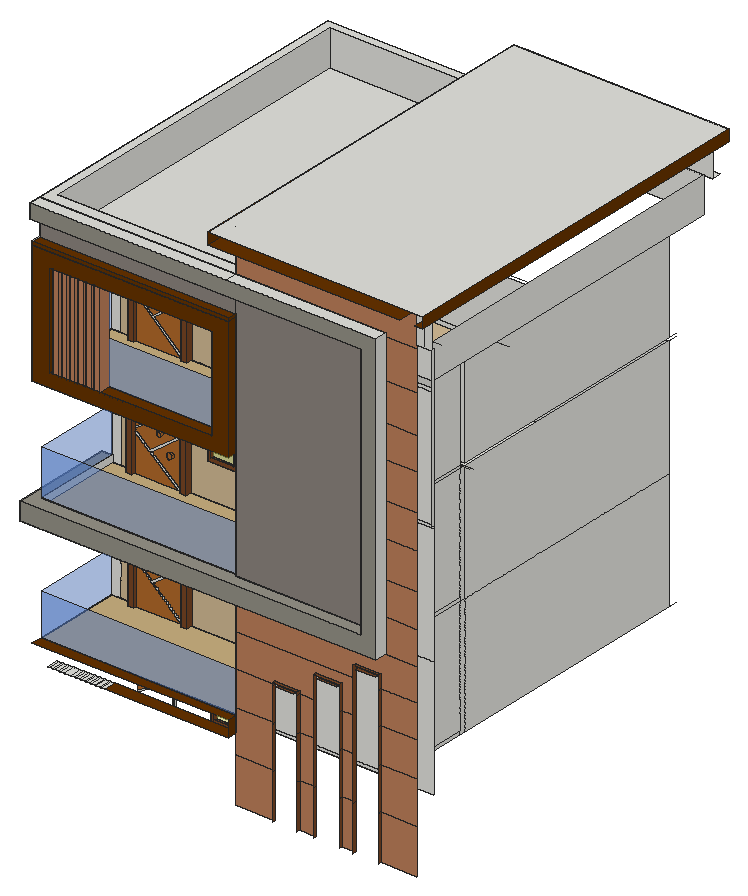
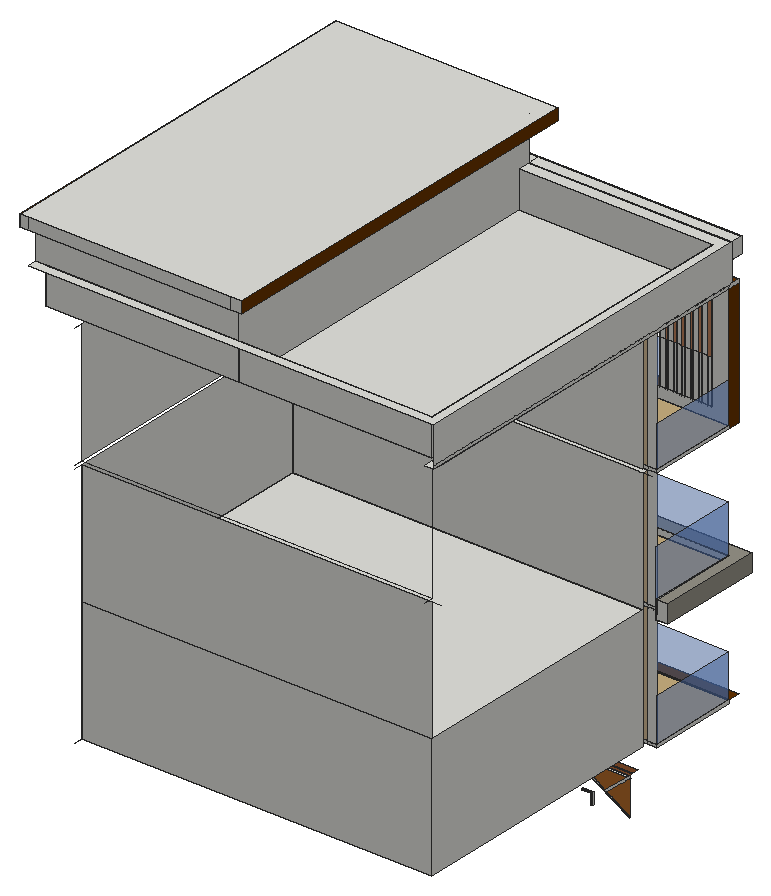
# SketchUp Ruby script. Lengths in inches.
U = 1.inch
M = Sketchup.active_model
def pt(a) = Geom::Point3d.new(a.map { |v| v * U })
def face(e, loops, mat)
  f = e.add_face(loops[0].map { |a| pt(a) })
  loops[1..].each { |l| e.add_face(l.map { |a| pt(a) }).erase! }
  f.material = f.back_material = mat if mat
  f
end
# faces: each face lists its corners as indices into pts; further lists are holes
def faces(e, pts, list, mat = nil) = list.each { |f| face(e, (f[0].is_a?(Array) ? f : [f]).map { |l| l.map { |i| pts[i] } }, mat) }
# xy, xz, yz: faces in a plane at the given z, y or x. An outline is a flat list of corners, or four numbers for a rectangle; further outlines are holes
def ring(l) = l.size == 4 ? [[l[0], l[1]], [l[2], l[1]], [l[2], l[3]], [l[0], l[3]]] : l.each_slice(2).to_a
def flat(e, list, mat, &to3) = list.each { |f| face(e, (f[0].is_a?(Array) ? f : [f]).map { |l| ring(l).map { |u, v| to3.(u, v) } }, mat) }
def xy(e, z, list, mat = nil) = flat(e, list, mat) { |x, y| [x, y, z] }
def xz(e, y, list, mat = nil) = flat(e, list, mat) { |x, z| [x, y, z] }
def yz(e, x, list, mat = nil) = flat(e, list, mat) { |y, z| [x, y, z] }
def lines(e, pts, list) = list.each { |a, b| e.add_line(pt(pts[a]), pt(pts[b])) }
# prism: a flat outline (further loops are holes) pulled along v
def prism(e, loops, v, mat = nil)
  f = face(e, loops, mat); d = Geom::Vector3d.new(v.map { |x| x * U })
  f.pushpull(f.normal.samedirection?(d) ? d.length : -d.length)
end
def box(e, o, s, mat = nil) = prism(e, [[o, [o[0] + s[0], o[1], o[2]], [o[0] + s[0], o[1] + s[1], o[2]], [o[0], o[1] + s[1], o[2]]]], [0, 0, s[2]], mat)
def at(x, y, z, deg = 0) = Geom::Transformation.translation(pt([x, y, z])) * Geom::Transformation.rotation(ORIGIN, Z_AXIS, deg.degrees)
def axes(o, x, y, z) = Geom::Transformation.new([*x, 0, *y, 0, *z, 0, *pt(o).to_a, 1])
def part(name) = M.definitions.add(name)
# library, detail: a bought-in or finely detailed component or shape, given as its bounding box
def library(name, o, s) = part(name).tap { |d| box(d.entities, o, s) }
def detail(e, o, s) = box(e.add_group.entities, o, s)
def put(e, d, t, mat = nil) = e.add_instance(d, t).tap { |i| i.material = mat if mat }
def group(e, t, mat = nil) = e.add_group.tap { |g| g.transformation = t; g.material = mat if mat }.entities
root = M.entities
M.materials.add("[Color C08]").color = [102, 51, 0]
M.materials.add("[Concrete Scored Jointless]").color = [140, 133, 127]
M.materials.add("[Formica Beige]").color = [211, 187, 149]
M.materials.add("[Formica Graystone]").color = [149, 146, 135]
M.materials.add("[Roofing Slate Tan]").color = [200, 175, 128]
M.materials.add("[Translucent Glass Blue]").color = [100, 149, 237]
M.materials["[Translucent Glass Blue]"].alpha = 0.5
M.materials.add("[Translucent Glass Gray]").color = [208, 209, 80]
M.materials["[Translucent Glass Gray]"].alpha = 0.5
M.materials.add("[Wood Bamboo]").color = [177, 105, 43]
M.materials.add("[Wood Veneer 01]").color = [120, 70, 37]
M.materials.add("[Wood Veneer 02]").color = [190, 128, 91]
prism(root,[[[75.279,109.4375,168.805],[75.279,109.4375,179.68],[85.654,109.4375,179.68],[85.654,109.4375,178.68],[76.654,109.4375,178.68],[76.654,109.4375,168.805]]],[0,-1,0])
xy(root,168.023,[[112.818,109.4375,168.881,112.4375]],"[Wood Veneer 01]")
xy(root,171.023,[[115.818,109.4375,135.318,112.4375],[138.318,109.4375,165.881,112.4375]],"[Wood Veneer 01]")
xy(root,207,[[39.278,109.4375,87.278,112.4375]])
xy(root,207,[[39.278,106.4375,87.278,109.4375]],"[Wood Veneer 01]")
xy(root,213,[[33.278,106.4375,93.278,112.4375]],"[Wood Veneer 01]")
xy(root,215.398,[[115.818,109.4375,135.318,112.4375],[138.318,109.4375,165.881,112.4375]],"[Wood Veneer 01]")
xy(root,218.398,[[112.818,109.4375,168.881,112.4375]],"[Wood Veneer 01]")
xy(root,230.125,[[43.358,12.4375,47.175,24.4375]])
xy(root,230.447,[[25.478,12.4375,27.42,24.4375],[27.42,12.4375,31.237,24.4375],[31.237,12.4375,32.733,24.4375],[32.733,12.4375,36.55,24.4375],[36.55,12.4375,38.045,24.4375],
  [38.045,12.4375,41.862,24.4375],[41.862,12.4375,48.67,24.4375],[48.67,12.4375,52.487,24.4375],[52.487,12.4375,53.983,24.4375],[53.983,12.4375,57.8,24.4375],
  [57.8,12.4375,59.295,24.4375],[59.295,12.4375,63.112,24.4375],[63.112,12.4375,64.358,24.4375],[64.358,12.4375,68.175,24.4375],[68.175,12.4375,69.42,24.4375],
  [69.42,12.4375,73.237,24.4375],[73.237,12.4375,74.483,24.4375],[74.483,12.4375,78.3,24.4375],[78.3,12.4375,79.545,24.4375],[79.545,12.4375,83.362,24.4375]])
xy(root,230.447,[[83.362,12.4375,207.712,24.4375]],"[Color C08]")
xy(root,243,[[19.125,118.4375,361.125,375.4375]])
xy(root,243,[[19.125,24.4375,361.125,112.4375]],"[Formica Beige]")
xy(root,246,[[207.712,21.4375,207.712,24.4375,10.125,24.4375],[30.863,106.4375,36.863,112.4375],[84.863,106.4375,90.863,112.4375],[36.863,109.4375,84.863,112.4375]])
xy(root,246,[[10.125,12.4375,207.712,12.4375,207.712,21.4375,10.125,24.4375]],"[Color C08]")
xy(root,246,[[10.125,24.4375,361.125,24.4375,361.125,112.4375,90.863,112.4375,90.863,106.4375,84.863,106.4375,84.863,109.4375,36.863,109.4375,36.863,106.4375,30.863,106.4375,30.863,112.4375,10.125,112.4375]],"[Roofing Slate Tan]")
xy(root,287.148,[[110.131,109.4375,166.193,112.4375]],"[Wood Veneer 01]")
xy(root,288.381,[[250.532,18.4375,269.237,21.4375]],"[Wood Veneer 01]")
xy(root,290.148,[[113.131,109.4375,135.318,112.4375],[138.318,109.4375,163.193,112.4375]],"[Wood Veneer 01]")
xy(root,291.381,[[247.532,18.4375,272.237,21.4375]],"[Wood Veneer 01]")
xy(root,309.988,[[291.733,18.4375,311.736,21.4375]],"[Wood Veneer 01]")
xy(root,312.988,[[288.733,18.4375,314.736,21.4375]],"[Wood Veneer 01]")
xy(root,330,[[36.863,106.4375,84.863,109.4375]])
xy(root,332.471,[[331.649,18.4375,351.153,21.4375]],"[Wood Veneer 01]")
xy(root,334.523,[[113.131,109.4375,135.318,112.4375],[138.318,109.4375,163.193,112.4375]],"[Wood Veneer 01]")
xy(root,335.471,[[328.649,18.4375,354.153,21.4375]],"[Wood Veneer 01]")
xy(root,336,[[30.863,106.4375,90.863,112.4375]],"[Wood Veneer 01]")
xy(root,337.523,[[110.131,109.4375,166.193,112.4375]],"[Wood Veneer 01]")
xy(root,354.75,[[0,9.4375,0,112.4375,10.785,112.4375,10.785,23.9375,207.712,23.9375,207.712,21.4375,343.389,21.4375,343.389,9.4375],[343.389,9.4375,358.6875,21.4375]],"[Formica Graystone]")
xy(root,363,[[19.125,118.4375,361.125,375.4375]])
xy(root,363,[[10.125,24.4375,361.125,112.4375]],"[Formica Beige]")
xy(root,366,[[29.633,106.4375,35.633,112.4375],[83.633,106.4375,89.633,112.4375],[35.633,109.4375,83.633,112.4375]])
xy(root,366,[[10.125,24.4375,361.125,24.4375,361.125,112.4375,89.633,112.4375,89.633,106.4375,83.633,106.4375,83.633,109.4375,35.633,109.4375,35.633,106.4375,29.633,106.4375,29.633,112.4375,10.125,112.4375]],"[Roofing Slate Tan]")
xy(root,372.201,[[0,9.4375,343.389,9.4375,343.389,21.4375,207.712,21.4375,207.712,23.9375,10.785,23.9375,10.785,112.4375,0,112.4375]],"[Formica Graystone]")
xy(root,403.273,[[109.068,109.4375,171.131,112.4375]])
xy(root,406.273,[[112.068,109.4375,135.318,112.4375],[138.318,109.4375,168.131,112.4375]],"[Wood Veneer 01]")
xy(root,450,[[35.633,106.4375,83.633,109.4375]])
xy(root,456,[[29.633,106.4375,89.633,112.4375]],"[Wood Veneer 01]")
xy(root,456.648,[[112.068,109.4375,135.318,112.4375],[138.318,109.4375,168.131,112.4375]],"[Wood Veneer 01]")
xy(root,459.648,[[109.068,109.4375,171.131,112.4375]],"[Wood Veneer 01]")
xy(root,483,[[19.125,112.4375,361.125,118.4375]])
xy(root,483,[[10.125,12.4375,207.712,24.4375]],"[Color C08]")
xy(root,483,[[10.125,24.4375,361.125,112.4375]],"[Formica Beige]")
xy(root,486,[[30.871,106.4375,36.871,112.4375],[84.871,106.4375,90.871,112.4375],[36.871,109.4375,84.871,112.4375]])
xy(root,486,[[10.125,24.4375,361.125,24.4375,361.125,112.4375,90.871,112.4375,90.871,106.4375,84.871,106.4375,84.871,109.4375,36.871,109.4375,36.871,106.4375,30.871,106.4375,30.871,112.4375,10.125,112.4375]],"[Roofing Slate Tan]")
xy(root,496.354,[[31.283,12.4375,37.045,24.4375],[37.045,12.4375,39.47,24.4375],[39.47,12.4375,45.233,24.4375],[45.233,12.4375,47.658,24.4375],[47.658,12.4375,53.42,24.4375],
  [53.42,12.4375,55.845,24.4375],[55.845,12.4375,61.608,24.4375],[61.608,12.4375,64.033,24.4375],[64.033,12.4375,69.795,24.4375],[69.795,12.4375,72.22,24.4375],
  [72.22,12.4375,77.983,24.4375]])
xy(root,496.354,[[27.41,12.4375,31.283,24.4375],[77.983,12.4375,190.722,24.4375]],"[Color C08]")
xy(root,525.398,[[110.131,109.4375,166.193,112.4375]],"[Wood Veneer 01]")
xy(root,528.398,[[113.131,109.4375,135.318,112.4375],[138.318,109.4375,163.193,112.4375]],"[Wood Veneer 01]")
xy(root,536.456,[[60.026,108.4375,74.714,109.4375]],"[Wood Bamboo]")
xy(root,540.894,[[60.026,108.4375,74.714,109.4375]],"[Wood Bamboo]")
xy(root,570,[[36.871,106.4375,84.871,109.4375]])
xy(root,572.773,[[113.131,109.4375,135.318,112.4375],[138.318,109.4375,163.193,112.4375]])
xy(root,575.773,[[110.131,109.4375,166.193,112.4375]])
xy(root,576,[[30.871,106.4375,90.871,112.4375]],"[Wood Veneer 01]")
xy(root,591.0625,[[27.41,12.4375,31.283,24.4375],[31.283,12.4375,37.045,24.4375],[37.045,12.4375,39.47,24.4375],[39.47,12.4375,45.233,24.4375],[45.233,12.4375,47.658,24.4375],
  [47.658,12.4375,53.42,24.4375],[53.42,12.4375,55.845,24.4375],[55.845,12.4375,61.608,24.4375],[61.608,12.4375,64.033,24.4375],[64.033,12.4375,69.795,24.4375],
  [69.795,12.4375,72.22,24.4375],[72.22,12.4375,77.983,24.4375]])
xy(root,591.0625,[[77.983,12.4375,190.722,24.4375]],"[Color C08]")
xy(root,606,[[10.125,12.4375,207.712,24.4375],[10.125,118.4375,19.125,375.4375],[10.125,375.4375,19.125,384.4375]])
xy(root,606,[[10.125,24.4375,361.125,112.4375]],"[Formica Beige]")
xy(root,609,[[10.125,21.4375,207.712,24.4375],[19.125,33.4375,207.712,375.4375]])
xy(root,609,[[10.125,12.4375,207.712,21.4375]],"[Color C08]")
xy(root,630.0625,[[10.125,9.4375,207.712,21.4375],[207.712,9.4375,343.389,21.4375]])
xy(root,645,[[10.125,9.4375,207.712,21.4375],[207.712,9.4375,358.6875,21.4375],[10.125,21.4375,207.712,21.4375,207.712,33.4375,19.125,33.4375,19.125,375.4375,405.5,375.4375,405.5,384.4375,10.125,384.4375]])
xy(root,676.624,[[207.712,21.4375,405.5,375.4375],[207.712,375.4375,405.5,385.625],[405.5,375.4375,413.3125,385.625]])
xy(root,676.624,[[196.462,0,196.462,385.625,207.712,385.625,207.712,21.4375,390.57,21.4375,390.57,0],[405.5,0,413.3125,375.4375]],"[Color C08]")
xy(root,688,[[196.462,0,413.3125,385.625]])
xz(root,9.4375,[[0,354.75,358.6875,354.75,358.6875,645,10.125,645,10.125,630.0625,343.389,630.0625,343.389,372.201,0,372.201]],"[Formica Graystone]")
xz(root,12.4375,[[[10.125,483,207.712,606],[27.41,496.354,190.722,591.0625]],[10.125,606,207.712,609]],"[Color C08]")
xz(root,12.4375,[[31.283,496.354,37.045,591.0625],[39.47,496.354,45.233,591.0625],[47.658,496.354,53.42,591.0625],[55.845,496.354,61.608,591.0625],[64.033,496.354,69.795,591.0625],
  [72.22,496.354,77.983,591.0625]],"[Wood Veneer 02]")
xz(root,21.4375,[[343.389,354.75,343.389,630.0625,10.125,630.0625,10.125,645,207.712,645,207.712,641.086,358.6875,641.086,358.6875,354.75],[207.712,354.75,343.389,372.201],[207.712,641.086,358.6875,645],[390.57,645,397.32,676.624],[397.32,645,405.5,676.624]])
xz(root,21.4375,[[207.712,372.201,343.389,630.0625],[10.125,609,207.712,630.0625]],"[Concrete Scored Jointless]")
xz(root,21.4375,[[207.712,165.318,247.532,210.382],[272.237,165.318,288.733,210.382],[314.736,165.318,328.649,210.382],[354.153,165.318,390.57,210.382],[207.712,210.382,247.532,253.461],
  [272.237,210.382,288.733,253.461],[314.736,210.382,328.649,253.461],[354.153,210.382,390.57,253.461],[207.712,253.461,247.532,288.381],[272.237,253.461,288.733,288.381],
  [314.736,253.461,328.649,288.381],[354.153,253.461,390.57,288.381],[207.712,288.381,247.532,288.381,247.532,291.381,272.237,291.381,272.237,288.381,288.733,288.381,288.733,312.988,314.736,312.988,314.736,288.381,328.649,288.381,328.649,321.566,207.712,321.566],[354.153,288.381,390.57,321.566],[207.712,321.566,328.649,321.566,328.649,335.471,354.153,335.471,354.153,321.566,390.57,321.566,390.57,354.75,207.712,354.75],
  [358.6875,354.75,390.57,388.211],[358.6875,388.211,390.57,421.672],[358.6875,421.672,390.57,458.887],[358.6875,458.887,390.57,493.388],[358.6875,493.388,390.57,530.159],
  [358.6875,530.159,390.57,563.208],[358.6875,563.208,390.57,601.74],[358.6875,601.74,390.57,641.086],[358.6875,641.086,390.57,641.086,390.57,676.624,207.712,676.624,207.712,645,358.6875,645]],"[Wood Veneer 02]")
xz(root,23.9375,[[10.785,354.75,207.712,372.201]])
xz(root,24.4375,[[10.125,243,207.712,246],[207.712,243,361.125,246],[361.125,243,405.5,363],[207.712,246,361.125,363],[10.125,363,207.712,366],
  [207.712,363,361.125,366],[361.125,363,405.5,483],[207.712,366,361.125,483],[10.125,483,192.347,486],[192.347,483,207.712,486],
  [207.712,483,361.125,486],[361.125,483,405.5,486],[[10.125,486,207.712,606],[27.41,496.354,190.722,591.0625]],[207.712,486,361.125,606],[361.125,486,405.5,606],
  [27.41,496.354,31.283,539.987],[31.283,496.354,37.045,539.987],[37.045,496.354,39.47,539.987],[39.47,496.354,45.233,539.987],[45.233,496.354,47.658,539.987],
  [47.658,496.354,53.42,539.987],[53.42,496.354,55.845,539.987],[55.845,496.354,61.608,539.987],[61.608,496.354,64.033,539.987],[64.033,496.354,69.795,539.987],
  [69.795,496.354,72.22,539.987],[72.22,496.354,77.983,539.987],[31.283,539.987,37.045,591.0625],[39.47,539.987,45.233,591.0625],[47.658,539.987,53.42,591.0625],
  [55.845,539.987,61.608,591.0625],[64.033,539.987,69.795,591.0625],[72.22,539.987,77.983,591.0625],[10.125,606,207.712,609],[207.712,606,361.125,609],
  [361.125,606,405.5,609]])
xz(root,24.4375,[[77.983,496.354,190.722,539.987]],"[Translucent Glass Blue]")
xz(root,33.4375,[[19.125,609,207.712,645],[207.712,609,361.125,645],[361.125,609,396.5,645]])
xz(root,106.4375,[[69.252,295.769,70.239,295.899,71.158,296.28,71.948,296.885,72.554,297.675,72.934,298.595,73.064,299.581,72.934,300.568,72.554,301.488,71.948,302.277,71.158,302.883,70.239,303.264,69.252,303.394,68.265,303.264,67.346,302.883,66.556,302.277,65.95,301.488,65.569,300.568,65.439,299.581,65.569,298.595,65.95,297.675,66.556,296.885,67.346,296.28,68.265,295.899],[72.635,392.462,75.125,393.899,75.125,396.774,72.635,398.212,70.145,396.774,70.145,393.899],[62.156,409.119,64.375,410.4,64.375,412.962,62.156,414.244,59.937,412.962,59.937,410.4]],"[Wood Bamboo]")
xz(root,106.4375,[[30.863,246,36.863,246,36.863,330,84.863,330,84.863,246,90.863,246,90.863,336,30.863,336],[29.633,366,35.633,366,35.633,450,83.633,450,83.633,366,89.633,366,89.633,456,29.633,456],[30.871,486,36.871,486,36.871,570,84.871,570,84.871,486,90.871,486,90.871,576,30.871,576]],"[Wood Veneer 01]")
xz(root,108.4375,[[60.026,536.456,74.714,540.894]],"[Wood Bamboo]")
xz(root,109.4375,[[39.278,169.997,87.278,198.612,87.278,200.487,63.278,186.179,39.278,207,39.278,204.447,61.534,185.14,39.278,171.872],[82.156,246,84.863,246,54.802,273.761,84.863,295.221,84.863,297.929,53.148,275.288,36.863,290.326,36.863,287.826],[36.863,290.326,84.863,327.9375,84.863,330,60.863,311.194,36.863,330,36.863,328.038,59.611,310.214,36.863,292.389],[80.508,366,83.633,366,52.949,391.49,83.633,414.459,83.633,416.795,51.408,392.77,35.633,405.875,35.633,403.279],[35.633,405.875,83.633,441.728,83.633,443.853,55.085,422.529,55.038,422.6,37.331,450,35.633,450,53.939,421.673,35.633,408],
  [83.192,486,84.871,486,54.524,513.678,84.871,536.456,84.871,538.848,53.477,514.632,36.871,529.777,36.871,528.246,37.756,527.439],[36.871,529.777,84.871,567.5625,84.871,570,61.594,551.676,36.871,570,36.871,567.9375,60.245,550.614,36.871,532.215]])
xz(root,109.4375,[[39.278,171.872,61.534,185.14,39.278,204.447],[63.278,186.179,87.278,200.487,87.278,207,39.278,207],[36.863,246,82.156,246,36.863,287.826],[84.863,246,84.863,295.221,54.802,273.761],[[53.148,275.288,84.863,297.929,84.863,327.9375,36.863,290.326],[69.252,295.769,68.265,295.899,67.346,296.28,66.556,296.885,65.95,297.675,65.569,298.595,65.439,299.581,65.569,300.568,65.95,301.488,66.556,302.277,67.346,302.883,68.265,303.264,69.252,303.394,70.239,303.264,71.158,302.883,71.948,302.277,72.554,301.488,72.934,300.568,73.064,299.581,72.934,298.595,72.554,297.675,71.948,296.885,71.158,296.28,70.239,295.899]],
  [36.863,292.389,59.611,310.214,36.863,328.038],[60.863,311.194,84.863,330,36.863,330],[35.633,366,80.508,366,35.633,403.279],[[83.633,366,83.633,414.459,52.949,391.49],[72.635,392.462,70.145,393.899,70.145,396.774,72.635,398.212,75.125,396.774,75.125,393.899]],[[51.408,392.77,83.633,416.795,83.633,441.728,35.633,405.875],[62.156,409.119,59.937,410.4,59.937,412.962,62.156,414.244,64.375,412.962,64.375,410.4]],
  [35.633,408,53.939,421.673,35.633,450],[55.085,422.529,83.633,443.853,83.633,450,37.331,450,55.038,422.6],[36.871,486,83.192,486,37.756,527.439,36.871,528.246],[84.871,486,84.871,536.456,54.524,513.678],[[53.477,514.632,84.871,538.848,84.871,567.5625,36.871,529.777],[60.026,536.456,74.714,540.894]],
  [36.871,532.215,60.245,550.614,36.871,567.9375],[61.594,551.676,84.871,570,36.871,570]],"[Wood Bamboo]")
xz(root,109.4375,[[[112.818,168.023,168.881,218.398],[138.318,171.023,165.881,215.398],[115.818,171.023,135.318,215.398]],[[110.131,287.148,166.193,337.523],[138.318,290.148,163.193,334.523],[113.131,290.148,135.318,334.523]],[[109.068,403.273,171.131,459.648],[138.318,406.273,168.131,456.648],[112.068,406.273,135.318,456.648]],[[110.131,525.398,166.193,575.773],[138.318,528.398,163.193,572.773],[113.131,528.398,135.318,572.773]]],"[Wood Veneer 01]")
xz(root,112.4375,[[10.125,243,19.125,246],[19.125,243,30.863,246],[30.863,243,90.863,246],[90.863,243,361.125,246],[10.125,246,19.125,246,19.125,363,10.785,363,10.785,354.75,10.125,354.75],
  [0,354.75,10.125,372.201],[10.125,354.75,10.785,363],[10.125,363,10.785,366],[10.785,363,19.125,366],[19.125,363,29.633,366],
  [29.633,363,89.633,366],[89.633,363,361.125,366],[10.125,366,10.785,372.201],[10.785,366,19.125,366,19.125,483,10.125,483,10.125,372.201,10.785,372.201],[10.125,483,19.125,486],
  [19.125,483,30.871,486],[30.871,483,90.871,486],[90.871,483,361.125,486],[10.125,486,19.125,606]])
xz(root,112.4375,[[[19.125,246,30.863,246,30.863,336,90.863,336,90.863,246,361.125,246,361.125,363,19.125,363],[110.131,287.148,166.193,337.523]],[[19.125,366,29.633,366,29.633,456,89.633,456,89.633,366,361.125,366,361.125,483,19.125,483],[109.068,403.273,171.131,459.648]],[[19.125,486,30.871,486,30.871,576,90.871,576,90.871,486,361.125,486,361.125,606,19.125,606],[110.131,525.398,166.193,575.773]]],"[Formica Beige]")
xz(root,112.4375,[[115.818,171.023,135.318,215.398],[138.318,171.023,165.881,215.398],[113.131,290.148,135.318,334.523],[138.318,290.148,163.193,334.523],[112.068,406.273,135.318,456.648],
  [138.318,406.273,168.131,456.648],[113.131,528.398,135.318,572.773],[138.318,528.398,163.193,572.773]],"[Translucent Glass Gray]")
xz(root,118.4375,[[19.125,243,361.125,363],[19.125,363,361.125,483],[19.125,486,361.125,606]])
xz(root,375.4375,[[19.125,243,361.125,363],[19.125,363,361.125,483],[19.125,609,207.712,645],[207.712,609,396.5,645],[207.712,645,405.5,676.624]])
xz(root,385.625,[[196.462,676.624,207.712,688],[207.712,676.624,405.5,688],[405.5,676.624,413.3125,688]])
yz(root,0,[[9.4375,354.75,112.4375,372.201]],"[Formica Graystone]")
yz(root,10.125,[[24.4375,243,112.4375,246],[24.4375,363,112.4375,366],[24.4375,483,112.4375,486],[12.4375,606,24.4375,609],[24.4375,606,384.4375,609],
  [21.4375,609,384.4375,645],[9.4375,630.0625,21.4375,645]])
yz(root,10.125,[[12.4375,483,24.4375,606]],"[Color C08]")
yz(root,10.125,[[24.4375,246,112.4375,288.381],[24.4375,486,112.4375,526.301]],"[Translucent Glass Blue]")
yz(root,10.785,[[23.9375,354.75,112.4375,372.201]])
yz(root,10.785,[[23.9375,372.201,112.4375,418.929]],"[Translucent Glass Blue]")
yz(root,19.125,[[118.4375,243,375.4375,363],[33.4375,609,375.4375,645]])
yz(root,27.41,[[12.4375,496.354,24.4375,591.0625]],"[Color C08]")
yz(root,29.633,[[106.4375,366,112.4375,456]],"[Wood Veneer 01]")
yz(root,30.863,[[106.4375,246,112.4375,336]],"[Wood Veneer 01]")
yz(root,30.871,[[106.4375,486,112.4375,576]],"[Wood Veneer 01]")
yz(root,31.283,[[12.4375,496.354,24.4375,591.0625]],"[Wood Veneer 02]")
yz(root,35.633,[[106.4375,366,109.4375,450]],"[Wood Veneer 01]")
yz(root,36.863,[[106.4375,246,109.4375,330]],"[Wood Veneer 01]")
yz(root,36.871,[[106.4375,486,109.4375,570]],"[Wood Veneer 01]")
yz(root,37.045,[[12.4375,496.354,24.4375,591.0625]],"[Wood Veneer 02]")
yz(root,39.47,[[12.4375,496.354,24.4375,591.0625]],"[Wood Veneer 02]")
yz(root,45.233,[[12.4375,496.354,24.4375,591.0625]],"[Wood Veneer 02]")
yz(root,47.658,[[12.4375,496.354,24.4375,591.0625]],"[Wood Veneer 02]")
yz(root,53.42,[[12.4375,496.354,24.4375,591.0625]],"[Wood Veneer 02]")
yz(root,55.845,[[12.4375,496.354,24.4375,591.0625]],"[Wood Veneer 02]")
yz(root,59.937,[[106.4375,410.4,109.4375,412.962]],"[Wood Bamboo]")
yz(root,60.026,[[108.4375,536.456,109.4375,540.894]],"[Wood Bamboo]")
yz(root,61.608,[[12.4375,496.354,24.4375,591.0625]],"[Wood Veneer 02]")
yz(root,64.033,[[12.4375,496.354,24.4375,591.0625]],"[Wood Veneer 02]")
yz(root,64.375,[[106.4375,410.4,109.4375,412.962]],"[Wood Bamboo]")
yz(root,69.795,[[12.4375,496.354,24.4375,591.0625]],"[Wood Veneer 02]")
yz(root,70.145,[[106.4375,393.899,109.4375,396.774]],"[Wood Bamboo]")
yz(root,72.22,[[12.4375,496.354,24.4375,591.0625]],"[Wood Veneer 02]")
yz(root,74.714,[[108.4375,536.456,109.4375,540.894]],"[Wood Bamboo]")
yz(root,75.125,[[106.4375,393.899,109.4375,396.774]],"[Wood Bamboo]")
yz(root,77.983,[[12.4375,496.354,24.4375,591.0625]],"[Wood Veneer 02]")
yz(root,83.633,[[106.4375,366,109.4375,450]],"[Wood Veneer 01]")
yz(root,84.863,[[106.4375,246,109.4375,330]],"[Wood Veneer 01]")
yz(root,84.871,[[106.4375,486,109.4375,570]],"[Wood Veneer 01]")
yz(root,89.633,[[106.4375,366,112.4375,456]],"[Wood Veneer 01]")
yz(root,90.863,[[106.4375,246,112.4375,336]],"[Wood Veneer 01]")
yz(root,90.871,[[106.4375,486,112.4375,576]],"[Wood Veneer 01]")
yz(root,109.068,[[109.4375,403.273,112.4375,459.648]],"[Wood Veneer 01]")
yz(root,110.131,[[109.4375,287.148,112.4375,337.523],[109.4375,525.398,112.4375,575.773]],"[Wood Veneer 01]")
yz(root,112.068,[[109.4375,406.273,112.4375,456.648]],"[Wood Veneer 01]")
yz(root,112.818,[[109.4375,168.023,112.4375,218.398]],"[Wood Veneer 01]")
yz(root,113.131,[[109.4375,290.148,112.4375,334.523],[109.4375,528.398,112.4375,572.773]],"[Wood Veneer 01]")
yz(root,115.818,[[109.4375,171.023,112.4375,215.398]],"[Wood Veneer 01]")
yz(root,135.318,[[109.4375,171.023,112.4375,215.398],[109.4375,290.148,112.4375,334.523],[109.4375,406.273,112.4375,456.648],[109.4375,528.398,112.4375,572.773]],"[Wood Veneer 01]")
yz(root,138.318,[[109.4375,171.023,112.4375,215.398],[109.4375,290.148,112.4375,334.523],[109.4375,406.273,112.4375,456.648],[109.4375,528.398,112.4375,572.773]],"[Wood Veneer 01]")
yz(root,163.193,[[109.4375,290.148,112.4375,334.523],[109.4375,528.398,112.4375,572.773]],"[Wood Veneer 01]")
yz(root,165.881,[[109.4375,171.023,112.4375,215.398]],"[Wood Veneer 01]")
yz(root,166.193,[[109.4375,287.148,112.4375,337.523],[109.4375,525.398,112.4375,575.773]])
yz(root,168.131,[[109.4375,406.273,112.4375,456.648]],"[Wood Veneer 01]")
yz(root,168.881,[[109.4375,168.023,112.4375,218.398]])
yz(root,171.131,[[109.4375,403.273,112.4375,459.648]],"[Wood Veneer 01]")
yz(root,190.722,[[12.4375,496.354,24.4375,591.0625]],"[Color C08]")
yz(root,196.462,[[0,676.624,385.625,688]],"[Color C08]")
yz(root,207.712,[[21.4375,230.447,24.4375,246],[[21.4375,246,21.4375,354.75,23.9375,354.75,23.9375,372.201,21.4375,372.201,21.4375,483,24.4375,483,24.4375,246],[21.571,288.49,21.604,288.492,21.634,288.504,21.661,288.522,21.682,288.548,21.696,288.577,21.701,288.609,21.698,288.642,21.687,288.672,21.669,288.699,21.643,288.72,21.614,288.734,21.582,288.739,21.549,288.736,21.519,288.725,21.492,288.706,21.471,288.681,21.457,288.652,21.452,288.62,21.455,288.587,21.466,288.557,21.485,288.53,21.51,288.509,21.539,288.495]],[21.571,288.49,21.539,288.495,21.51,288.509,21.485,288.53,21.466,288.557,21.455,288.587,21.452,288.62,21.457,288.652,21.471,288.681,21.492,288.706,21.519,288.725,21.549,288.736,21.582,288.739,21.614,288.734,21.643,288.72,21.669,288.699,21.687,288.672,21.698,288.642,21.701,288.609,21.696,288.577,21.682,288.548,21.661,288.522,21.634,288.504,21.604,288.492],[21.4375,354.75,23.9375,372.201],[21.4375,483,24.4375,606],
  [21.4375,606,24.4375,609],[33.4375,609,33.4375,645,21.4375,645,21.4375,676.624,375.4375,676.624,375.4375,609]])
yz(root,207.712,[[12.4375,230.447,21.4375,246],[12.4375,483,21.4375,606],[12.4375,606,21.4375,609]],"[Color C08]")
yz(root,247.532,[[18.4375,165.318,21.4375,210.382],[18.4375,210.382,21.4375,253.461],[18.4375,253.461,21.4375,288.381],[18.4375,288.381,21.4375,291.381]],"[Wood Veneer 01]")
yz(root,272.237,[[18.4375,165.318,21.4375,210.382],[18.4375,210.382,21.4375,253.461],[18.4375,253.461,21.4375,288.381],[18.4375,288.381,21.4375,291.381]],"[Wood Veneer 01]")
yz(root,288.733,[[18.4375,165.318,21.4375,210.382],[18.4375,210.382,21.4375,312.988]],"[Wood Veneer 01]")
yz(root,314.736,[[18.4375,165.318,21.4375,210.382],[18.4375,210.382,21.4375,253.461],[18.4375,253.461,21.4375,288.381],[18.4375,288.381,21.4375,312.988]],"[Wood Veneer 01]")
yz(root,328.649,[[18.4375,165.318,21.4375,210.382],[18.4375,210.382,21.4375,335.471]],"[Wood Veneer 01]")
yz(root,343.389,[[9.4375,372.201,21.4375,630.0625]],"[Formica Graystone]")
yz(root,354.153,[[18.4375,165.318,21.4375,210.382],[18.4375,210.382,21.4375,253.461],[18.4375,253.461,21.4375,288.381],[18.4375,288.381,21.4375,321.566],[18.4375,321.566,21.4375,335.471]],"[Wood Veneer 01]")
yz(root,358.6875,[[9.4375,354.75,21.4375,645]])
yz(root,361.125,[[24.4375,243,33.4375,246],[33.4375,243,112.4375,246],[112.4375,243,118.4375,363],[118.4375,243,375.4375,363],[24.4375,246,112.4375,363],
  [24.4375,363,112.4375,366],[112.4375,363,118.4375,483],[118.4375,363,375.4375,483],[24.4375,366,112.4375,483],[24.4375,483,112.4375,486],
  [24.4375,486,112.4375,606],[118.4375,486,375.4375,606]])
yz(root,396.5,[[33.4375,609,375.4375,645]])
yz(root,405.5,[[21.4375,486,24.4375,645]])
yz(root,413.3125,[[0,676.624,385.625,688]],"[Color C08]")
p = [[10.125,24.4375,246],[207.712,21.4375,246],[207.712,21.4375,253.461],[207.712,21.4375,288.381],[10.125,24.4375,288.381],[68.265,109.4375,295.899],
  [69.252,109.4375,295.769],[69.252,106.4375,295.769],[68.265,106.4375,295.899],[70.239,109.4375,295.899],[70.239,106.4375,295.899],[67.346,109.4375,296.28],
  [67.346,106.4375,296.28],[71.158,109.4375,296.28],[71.158,106.4375,296.28],[66.556,109.4375,296.885],[66.556,106.4375,296.885],[71.948,109.4375,296.885],
  [71.948,106.4375,296.885],[65.95,109.4375,297.675],[65.95,106.4375,297.675],[72.554,109.4375,297.675],[72.554,106.4375,297.675],[65.569,109.4375,298.595],
  [65.569,106.4375,298.595],[72.934,109.4375,298.595],[72.934,106.4375,298.595],[65.439,109.4375,299.581],[65.439,106.4375,299.581],[73.064,109.4375,299.581],
  [73.064,106.4375,299.581],[65.569,109.4375,300.568],[65.569,106.4375,300.568],[72.934,109.4375,300.568],[72.934,106.4375,300.568],[65.95,109.4375,301.488],
  [65.95,106.4375,301.488],[72.554,109.4375,301.488],[72.554,106.4375,301.488],[66.556,109.4375,302.277],[66.556,106.4375,302.277],[71.948,109.4375,302.277],
  [71.948,106.4375,302.277],[67.346,109.4375,302.883],[67.346,106.4375,302.883],[71.158,109.4375,302.883],[71.158,106.4375,302.883],[68.265,109.4375,303.264],
  [68.265,106.4375,303.264],[70.239,109.4375,303.264],[70.239,106.4375,303.264],[69.252,109.4375,303.394],[69.252,106.4375,303.394],[10.785,23.9375,372.201],
  [10.785,23.9375,418.929],[207.712,24.4375,418.929],[207.712,24.4375,372.201],[70.145,109.4375,393.899],[72.635,109.4375,392.462],[72.635,106.4375,392.462],
  [70.145,106.4375,393.899],[75.125,109.4375,393.899],[75.125,106.4375,393.899],[72.635,109.4375,398.212],[70.145,109.4375,396.774],[70.145,106.4375,396.774],
  [72.635,106.4375,398.212],[75.125,109.4375,396.774],[75.125,106.4375,396.774],[59.937,109.4375,410.4],[62.156,109.4375,409.119],[62.156,106.4375,409.119],
  [59.937,106.4375,410.4],[64.375,109.4375,410.4],[64.375,106.4375,410.4],[62.156,109.4375,414.244],[59.937,109.4375,412.962],[59.937,106.4375,412.962],
  [62.156,106.4375,414.244],[64.375,109.4375,412.962],[64.375,106.4375,412.962],[361.125,375.4375,243],[361.125,384.4375,243],[361.125,375.4375,483],
  [361.125,384.4375,483],[361.125,118.4375,483],[370.125,118.4375,483],[19.125,375.4375,483],[10.125,375.4375,483],[19.125,118.4375,483],
  [10.125,118.4375,483],[361.125,112.4375,486],[370.125,112.4375,486],[361.125,375.4375,486],[361.125,384.4375,486],[19.125,375.4375,486],
  [19.125,384.4375,486],[19.125,375.4375,606],[361.125,375.4375,606],[361.125,384.4375,606],[37.872,109.4375,205.667],[39.278,109.4375,204.447],
  [35.723,109.4375,328.931],[36.863,109.4375,328.038],[82.156,109.4375,246],[84.863,109.4375,243.5],[54.796,109.4375,273.757],[54.802,109.4375,273.761],
  [84.863,109.4375,295.221],[86.511,109.4375,296.398],[36.732,109.4375,450.927],[37.331,109.4375,450],[32.508,109.4375,405.875],[35.633,109.4375,403.279],
  [83.192,109.4375,486],[85.756,109.4375,483.662],[84.871,109.4375,536.456],[86.352,109.4375,537.599],[361.125,24.4375,609],[361.125,24.4375,645],
  [361.125,33.4375,645],[207.712,21.4375,676.624],[207.712,21.4375,688],[396.5,33.4375,645],[405.5,33.4375,645],[361.125,118.4375,606],
  [405.5,118.4375,606]]
faces(root,p,[[0,1,2,3,4],[53,54,55,56]],"[Translucent Glass Blue]")
faces(root,p,[[5,6,7,8],[6,9,10,7],[11,5,8,12],[9,13,14,10],[15,11,12,16],[13,17,18,14],[19,15,16,20],[17,21,22,18],
  [23,19,20,24],[21,25,26,22],[27,23,24,28],[25,29,30,26],[31,27,28,32],[29,33,34,30],[35,31,32,36],[33,37,38,34],
  [39,35,36,40],[37,41,42,38],[43,39,40,44],[41,45,46,42],[47,43,44,48],[45,49,50,46],[51,47,48,52],[49,51,52,50],
  [57,58,59,60],[58,61,62,59],[63,64,65,66],[67,63,66,68],[69,70,71,72],[70,73,74,71],[75,76,77,78],[79,75,78,80]],"[Wood Bamboo]")
lines(root,p,[[81,82],[83,84],[85,86],[87,88],[89,90],[91,92],[93,94],[95,96],[93,95],[95,97],[98,99],[100,101],
  [102,103],[104,105],[106,107],[108,109],[110,111],[112,113],[114,115],[116,117],[118,119],[120,119],[121,122],[123,124],
  [125,126]])
